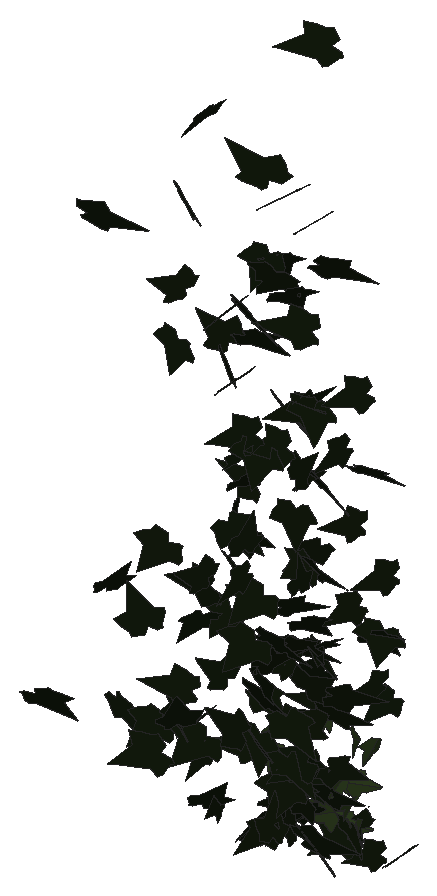
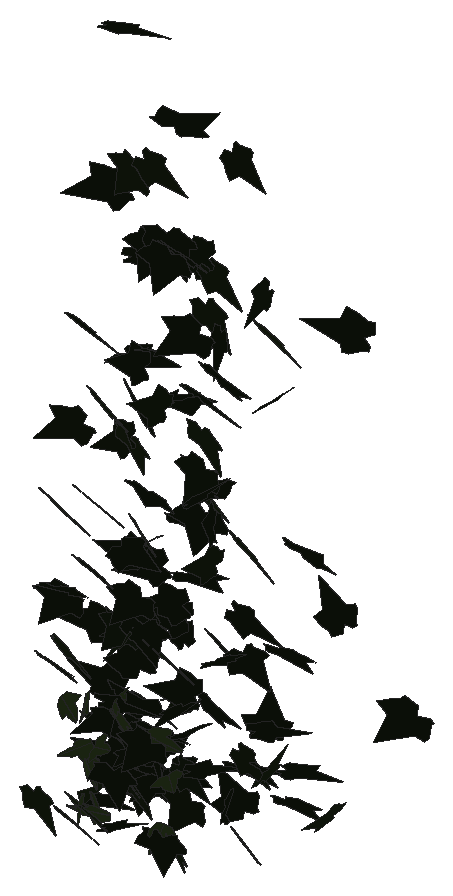
# SketchUp Ruby script. Lengths in inches.
U = 1.inch
M = Sketchup.active_model
def pt(a) = Geom::Point3d.new(a.map { |v| v * U })
def face(e, loops, mat)
  f = e.add_face(loops[0].map { |a| pt(a) })
  loops[1..].each { |l| e.add_face(l.map { |a| pt(a) }).erase! }
  f.material = f.back_material = mat if mat
  f
end
# faces: each face lists its corners as indices into pts; further lists are holes
def faces(e, pts, list, mat = nil) = list.each { |f| face(e, (f[0].is_a?(Array) ? f : [f]).map { |l| l.map { |i| pts[i] } }, mat) }
# xy, xz, yz: faces in a plane at the given z, y or x. An outline is a flat list of corners, or four numbers for a rectangle; further outlines are holes
def ring(l) = l.size == 4 ? [[l[0], l[1]], [l[2], l[1]], [l[2], l[3]], [l[0], l[3]]] : l.each_slice(2).to_a
def flat(e, list, mat, &to3) = list.each { |f| face(e, (f[0].is_a?(Array) ? f : [f]).map { |l| ring(l).map { |u, v| to3.(u, v) } }, mat) }
def xy(e, z, list, mat = nil) = flat(e, list, mat) { |x, y| [x, y, z] }
def xz(e, y, list, mat = nil) = flat(e, list, mat) { |x, z| [x, y, z] }
def yz(e, x, list, mat = nil) = flat(e, list, mat) { |y, z| [x, y, z] }
def lines(e, pts, list) = list.each { |a, b| e.add_line(pt(pts[a]), pt(pts[b])) }
# prism: a flat outline (further loops are holes) pulled along v
def prism(e, loops, v, mat = nil)
  f = face(e, loops, mat); d = Geom::Vector3d.new(v.map { |x| x * U })
  f.pushpull(f.normal.samedirection?(d) ? d.length : -d.length)
end
def box(e, o, s, mat = nil) = prism(e, [[o, [o[0] + s[0], o[1], o[2]], [o[0] + s[0], o[1] + s[1], o[2]], [o[0], o[1] + s[1], o[2]]]], [0, 0, s[2]], mat)
def at(x, y, z, deg = 0) = Geom::Transformation.translation(pt([x, y, z])) * Geom::Transformation.rotation(ORIGIN, Z_AXIS, deg.degrees)
def axes(o, x, y, z) = Geom::Transformation.new([*x, 0, *y, 0, *z, 0, *pt(o).to_a, 1])
def part(name) = M.definitions.add(name)
# library, detail: a bought-in or finely detailed component or shape, given as its bounding box
def library(name, o, s) = part(name).tap { |d| box(d.entities, o, s) }
def detail(e, o, s) = box(e.add_group.entities, o, s)
def put(e, d, t, mat = nil) = e.add_instance(d, t).tap { |i| i.material = mat if mat }
def group(e, t, mat = nil) = e.add_group.tap { |g| g.transformation = t; g.material = mat if mat }.entities
root = M.entities
M.materials.add("1026 AP 7946 SUNNY SIDE UP").color = [254, 231, 186]
M.materials.add("efeu1").color = [18, 25, 13]
M.materials.add("efeu2").color = [43, 57, 29]
c1 = part("ivyleaf_9")
p = [[1.54,2.16,1.25],[1.36,2.04,1.19],[-0.21,0.99,0.68],[-0.71,1.11,0.82],[-0.85,0.86,0.67],[-0.8,0.17,0.21],
  [-0.9,-0.01,0.1],[-0.67,-0.16,-0.02],[-0.08,-0.08,-0.05],[-0.03,-0.6,-0.4],[0.65,-0.88,-0.66],[0.83,-0.6,-0.49],
  [1.29,-0.42,-0.43],[1.8125,-0.07,-0.26],[1.21,0.44,0.15]]
faces(c1.entities,p,[[0,1,2,3,4,5,6,7,8,9,10,11,12,13,14]],"efeu1")
c2 = part("ivyleaf_10")
p = [[0,0.5,-0.03],[-0.0625,2.02,-0.43],[-0.19,2.01,-0.46],[-0.54,1.05,-0.29],[-0.52,0.625,-0.18],[-0.83,0.76,-0.28],
  [-1.16,0.64,-0.33],[-1.15,0.33,-0.24],[-0.77,-0.39,0.02],[-0.3,-0.51,0.16],[0.04,-0.48,0.23],[-0.02,2.01,-0.4375],
  [-0.06,2.01,-0.43],[0.04,-0.49,0.23],[0.67,-0.49,0.14],[1.38,0.36,-0.2],[1.375,0.51,-0.24],[0.81,0.65,-0.19],
  [0.62,0.59,-0.15],[0.6,1.09,-0.28],[0.5,1.23,-0.31]]
faces(c2.entities,p,[[0,1,2,3,4,5,6,7,8,9,10],[11,12,0,13,14,15,16,17,18,19,20]],"efeu2")
put(root,c1,axes([88.35,210.79,309.8125],[0.40505,-0.04361,0.36592],[0.56374,-0.08431,-0.26046],[0.15951,0.4087,-0.00867]),"1026 AP 7946 SUNNY SIDE UP")
put(root,c1,axes([89.35,207.07,295.36],[0.64023,0.15949,0.07493],[0.1307,-0.00845,-0.43669],[-0.26364,0.38312,-0.03454]),"1026 AP 7946 SUNNY SIDE UP")
put(root,c1,axes([89.51,210.67,293.62],[0.33265,-0.3478,-0.06127],[-0.00599,0.05837,-0.4257],[0.59711,0.19435,0.02986]),"1026 AP 7946 SUNNY SIDE UP")
put(root,c1,axes([90.67,211.54,299.03],[-0.62378,-0.1104,-0.03038],[0.06307,-0.03056,-0.40897],[0.1823,-0.36718,0.03755]),"1026 AP 7946 SUNNY SIDE UP")
put(root,c1,axes([90.63,208.78,298.75],[0.37595,0.32286,0.16484],[-0.18086,-0.10816,0.41679],[0.57645,-0.24449,0.02326]),"1026 AP 7946 SUNNY SIDE UP")
put(root,c1,axes([91.16,210.62,293.51],[-0.60289,-0.11549,0.01814],[-0.01057,-0.04023,-0.39849],[0.19826,-0.35335,0.03392]),"1026 AP 7946 SUNNY SIDE UP")
put(root,c1,axes([90.91,211.92,310.875],[0.49161,-0.16259,-0.24472],[-0.33845,0.10746,-0.35405],[0.3308,0.35158,0.00145]),"1026 AP 7946 SUNNY SIDE UP")
put(root,c1,axes([92.09,210.57,308.67],[-0.32947,0.31868,0.18492],[-0.23943,0.10907,-0.39308],[-0.56322,-0.23279,0.05893]),"1026 AP 7946 SUNNY SIDE UP")
put(root,c1,axes([91.61,210.9,306.55],[-0.14068,-0.35132,0.18544],[-0.04585,-0.17619,-0.38866],[0.66684,-0.08623,0.0124]),"1026 AP 7946 SUNNY SIDE UP")
put(root,c1,axes([92.28,209.15,293.47],[-0.54582,-0.12194,0.24605],[-0.3373,-0.12463,-0.36761],[0.28879,-0.37604,0.03568]),"1026 AP 7946 SUNNY SIDE UP")
put(root,c1,axes([92.07,211.68,292.41],[-0.48303,0.0833,-0.21493],[0.30168,-0.10429,-0.31575],[-0.21537,-0.33291,0.03974]),"1026 AP 7946 SUNNY SIDE UP")
put(root,c1,axes([92.47,210.33,295.18],[-0.31833,-0.00367,0.34467],[-0.52272,-0.10696,-0.19479],[0.15992,-0.35694,0.0494]),"1026 AP 7946 SUNNY SIDE UP")
put(root,c1,axes([92.02,210.6,293.96],[0.2802,-0.33926,-0.16995],[0.14409,-0.13013,0.40164],[-0.61607,-0.18474,0.01664]),"1026 AP 7946 SUNNY SIDE UP")
put(root,c1,axes([92.5,211.39,314.59],[-0.25235,0.27953,-0.28675],[0.14937,-0.25899,-0.34068],[-0.6444,-0.1695,0.03333]),"1026 AP 7946 SUNNY SIDE UP")
put(root,c1,axes([93.125,210.47,298.9],[-0.1617,0.01914,-0.41463],[-0.62963,-0.1217,0.08947],[-0.19346,0.38007,0.05539]),"1026 AP 7946 SUNNY SIDE UP")
put(root,c1,axes([92.81,210.56,297.71],[-0.00773,0.25127,-0.29953],[0.02589,-0.28273,-0.2729],[-0.642,-0.01443,-0.0074]),"1026 AP 7946 SUNNY SIDE UP")
put(root,c1,axes([93.17,211.3,306.93],[-0.08552,0.21206,0.37198],[-0.40306,0.2658,-0.20851],[-0.55633,-0.22517,0.09388]),"1026 AP 7946 SUNNY SIDE UP")
put(root,c1,axes([92.94,210.54,294.39],[-0.30718,0.25629,-0.20111],[0.11929,-0.18244,-0.33557],[-0.52952,-0.18978,0.04107]),"1026 AP 7946 SUNNY SIDE UP")
put(root,c1,axes([93.12,210.28,293.81],[-0.63395,-0.18201,0.03387],[-0.02398,-0.04835,-0.44366],[0.31341,-0.37187,0.03458]),"1026 AP 7946 SUNNY SIDE UP")
put(root,c1,axes([92.86,209.33,294.64],[0.4081,0.18786,0.28022],[-0.38447,-0.12943,0.32339],[0.38422,-0.32905,0.02597]),"1026 AP 7946 SUNNY SIDE UP")
put(root,c1,axes([93.51,207.04,299.23],[-0.67509,0.05875,-0.1237],[-0.18899,0.0409,0.43023],[0.11493,0.41232,-0.01913]),"1026 AP 7946 SUNNY SIDE UP")
put(root,c1,axes([93.16,211.38,297.73],[-0.31473,-0.29135,0.1333],[-0.06955,-0.12542,-0.37],[0.53593,-0.18737,0.03027]),"1026 AP 7946 SUNNY SIDE UP")
put(root,c1,axes([94.21,209,300.21],[-0.357,0.312,0.16237],[-0.16064,0.1141,-0.40096],[-0.56346,-0.23021,0.01144]),"1026 AP 7946 SUNNY SIDE UP")
put(root,c1,axes([93.57,209.68,291.99],[0.46659,0.25463,0.09948],[-0.14749,-0.03761,0.39926],[0.43383,-0.28664,0.02875]),"1026 AP 7946 SUNNY SIDE UP")
put(root,c1,axes([94.28,211.06,293.57],[-0.31836,-0.04355,0.33102],[-0.44932,-0.17038,-0.19959],[0.28298,-0.31952,0.0555]),"1026 AP 7946 SUNNY SIDE UP")
put(root,c1,axes([94.02,210.48,301.42],[-0.00216,-0.00823,0.43714],[0.20849,0.38953,0.01425],[-0.66139,0.12282,0.00306]),"1026 AP 7946 SUNNY SIDE UP")
put(root,c1,axes([93.89,210.03,292.07],[0.01141,-0.15424,-0.34654],[0.38309,-0.24735,0.12856],[-0.46903,-0.20578,0.09658]),"1026 AP 7946 SUNNY SIDE UP")
put(root,c1,axes([94.26,211.18,302.47],[-0.10473,-0.37314,-0.06699],[0.02257,-0.06059,0.40332],[-0.64055,0.05887,0.02517]),"1026 AP 7946 SUNNY SIDE UP")
put(root,c1,axes([94.27,209.82,307.33],[0.39042,-0.11108,-0.3503],[-0.5211,0.11097,-0.27099],[0.26421,0.38301,-0.01684]),"1026 AP 7946 SUNNY SIDE UP")
put(root,c1,axes([94.68,209.34,296.8125],[-0.22476,0.25202,0.28839],[-0.26401,0.21756,-0.3004],[-0.56335,-0.2025,0.02572]),"1026 AP 7946 SUNNY SIDE UP")
put(root,c1,axes([94.67,209.76,309.32],[-0.29723,0.30615,-0.21559],[0.10562,-0.19955,-0.37805],[-0.61682,-0.18169,0.03915]),"1026 AP 7946 SUNNY SIDE UP")
put(root,c1,axes([94.75,210.04,304.08],[-0.14315,0.38325,0.09427],[-0.06269,0.07682,-0.41855],[-0.66274,-0.09005,0.01923]),"1026 AP 7946 SUNNY SIDE UP")
put(root,c1,axes([94.07,210.38,300.1],[0.41419,-0.30856,0.10071],[0.07029,-0.09208,-0.42165],[0.54512,0.24633,-0.02216]),"1026 AP 7946 SUNNY SIDE UP")
put(root,c1,axes([94.49,210.32,303.06],[0.25798,0.33484,0.1589],[0.13227,0.12263,-0.39144],[-0.60448,0.16974,-0.01784]),"1026 AP 7946 SUNNY SIDE UP")
put(root,c1,axes([95.04,209.6,294.95],[-0.38704,0.00442,-0.35394],[-0.561,0.01157,0.24428],[0.02043,0.40148,0.00246]),"1026 AP 7946 SUNNY SIDE UP")
put(root,c1,axes([94.39,210.75,307.75],[0.58515,0.17168,0.13315],[0.19264,0.04603,-0.41152],[-0.30135,0.36279,-0.00452]),"1026 AP 7946 SUNNY SIDE UP")
put(root,c1,axes([94.68,210.08,301.43],[0.53247,0.18753,-0.15731],[-0.19567,-0.09774,-0.39184],[-0.35687,0.33339,-0.01987]),"1026 AP 7946 SUNNY SIDE UP")
put(root,c1,axes([95.05,211.03,290.97],[-0.24199,0.03498,-0.35985],[-0.49635,0.17113,0.15401],[0.28918,0.323,-0.0368]),"1026 AP 7946 SUNNY SIDE UP")
put(root,c1,axes([94.82,211.77,291.48],[0.36631,0.21053,-0.16052],[-0.16655,-0.11783,-0.32404],[-0.40885,0.23663,-0.01181]),"1026 AP 7946 SUNNY SIDE UP")
put(root,c2,axes([94.78,211.54,293.41],[0.22873,0.29279,-0.13915],[-0.06439,-0.12959,-0.34631],[-0.54265,0.13879,-0.01756]),"1026 AP 7946 SUNNY SIDE UP")
put(root,c1,axes([94.83,211.16,310.5],[-0.56283,-0.10998,-0.19496],[0.34668,-0.07901,-0.35084],[0.09346,-0.36923,0.1273]),"1026 AP 7946 SUNNY SIDE UP")
put(root,c1,axes([95.36,209.8,305.13],[-0.63491,0.15895,0.08712],[-0.14945,-0.00531,-0.43318],[-0.26191,-0.3823,0.03598]),"1026 AP 7946 SUNNY SIDE UP")
put(root,c1,axes([94.69,211.09,295.55],[0.13833,-0.28208,-0.24444],[-0.016,0.22856,-0.30773],[0.61193,0.06974,0.04721]),"1026 AP 7946 SUNNY SIDE UP")
put(root,c1,axes([94.96,211.28,310.34],[0.37038,0.32602,0.01366],[0.03741,-0.00453,-0.41945],[-0.55236,0.2183,-0.01925]),"1026 AP 7946 SUNNY SIDE UP")
put(root,c1,axes([94.81,209.38,302.11],[0.0867,-0.20404,-0.38713],[-0.06738,0.35759,-0.21866],[0.69765,0.05989,0.027]),"1026 AP 7946 SUNNY SIDE UP")
put(root,c2,axes([95.35,211.58,294.55],[0.21827,0.15991,-0.30184],[-0.428,-0.1447,-0.21144],[-0.35066,0.27616,0.07019]),"1026 AP 7946 SUNNY SIDE UP")
put(root,c2,axes([95.06,211.5,291.55],[-0.199,-0.27359,-0.20013],[0.1675,0.15653,-0.31537],[0.53342,-0.15122,0.02437]),"1026 AP 7946 SUNNY SIDE UP")
put(root,c1,axes([94.98,210.59,294.39],[-0.14677,-0.39406,0.07336],[0.02204,-0.07807,-0.43189],[0.68017,-0.0825,0.02982]),"1026 AP 7946 SUNNY SIDE UP")
put(root,c1,axes([95.46,208.95,307.47],[-0.17999,0.38931,-0.09475],[0.0238,-0.09314,-0.43312],[-0.67927,-0.10642,0.00993]),"1026 AP 7946 SUNNY SIDE UP")
put(root,c1,axes([95.64,210.13,313.875],[0.08829,0.12375,0.42573],[-0.6964,0.07519,0.03357],[-0.10562,-0.39231,0.1345]),"1026 AP 7946 SUNNY SIDE UP")
put(root,c1,axes([94.67,210.64,295.74],[0.48118,-0.18203,0.25205],[0.30577,-0.15797,-0.36151],[0.40615,0.33458,-0.02646]),"1026 AP 7946 SUNNY SIDE UP")
put(root,c1,axes([95.15,211.96,294.58],[0.54043,0.16246,0.00292],[0.02063,-0.02247,-0.38198],[-0.27502,0.31757,-0.02291]),"1026 AP 7946 SUNNY SIDE UP")
put(root,c1,axes([94.96,209.61,309.53],[0.54959,-0.23504,0.1061],[0.10894,-0.08502,-0.42829],[0.4212,0.32868,-0.02767]),"1026 AP 7946 SUNNY SIDE UP")
put(root,c1,axes([95.66,210.51,310.45],[0.35833,0.13459,-0.34297],[-0.45301,-0.18048,-0.27047],[-0.38207,0.34021,-0.00097]),"1026 AP 7946 SUNNY SIDE UP")
put(root,c1,axes([95.4,209.82,291.63],[0.28304,0.33113,0.1889],[0.13305,0.15325,-0.39477],[-0.61938,0.18424,0.00152]),"1026 AP 7946 SUNNY SIDE UP")
put(root,c1,axes([95.96,210.95,297.1],[-0.54413,0.2458,0.04579],[-0.10667,-0.01746,-0.42911],[-0.40894,-0.3225,0.051]),"1026 AP 7946 SUNNY SIDE UP")
put(root,c1,axes([95.09,211.48,305.36],[0.39573,-0.27888,0.19115],[0.16185,-0.1572,-0.39043],[0.54182,0.25064,-0.02298]),"1026 AP 7946 SUNNY SIDE UP")
put(root,c1,axes([95.76,208.9,301.83],[-0.46951,0.2629,-0.12032],[-0.12898,0.0881,0.40959],[0.4703,0.28662,-0.00779]),"1026 AP 7946 SUNNY SIDE UP")
put(root,c1,axes([95.92,211.14,313.07],[-0.34268,0.26206,-0.23595],[0.02122,-0.25365,-0.33356],[-0.58463,-0.16281,0.1262]),"1026 AP 7946 SUNNY SIDE UP")
put(root,c1,axes([95.67,209.79,304.69],[-0.34234,-0.34354,-0.01321],[0.0411,-0.00511,-0.42581],[0.58189,-0.20176,0.0223]),"1026 AP 7946 SUNNY SIDE UP")
put(root,c1,axes([95.92,209.57,292.47],[-0.28818,0.2543,-0.25059],[0.16828,-0.21783,-0.32876],[-0.56606,-0.19422,0.02984]),"1026 AP 7946 SUNNY SIDE UP")
put(root,c1,axes([95.93,209.11,298.59],[-0.5587,-0.23379,0.0543],[-0.04548,-0.05489,-0.43185],[0.40468,-0.32894,0.02643]),"1026 AP 7946 SUNNY SIDE UP")
put(root,c1,axes([96.1,210.375,304.71],[-0.29778,-0.11327,0.3473],[-0.36446,-0.25033,-0.22038],[0.45845,-0.27259,0.05039]),"1026 AP 7946 SUNNY SIDE UP")
put(root,c1,axes([96.04,211.15,297.76],[0.24108,0.26625,-0.21466],[-0.18017,-0.17445,-0.32533],[-0.5401,0.17704,0.01271]),"1026 AP 7946 SUNNY SIDE UP")
put(root,c1,axes([96.1,208.5,301.17],[-0.53534,0.18536,-0.20246],[0.24953,-0.12655,-0.39201],[-0.37743,-0.34658,0.028]),"1026 AP 7946 SUNNY SIDE UP")
put(root,c1,axes([96.12,211.95,300.64],[-0.08308,0.09831,-0.38832],[0.05864,-0.36434,-0.11541],[-0.63736,-0.04634,0.04]),"1026 AP 7946 SUNNY SIDE UP")
put(root,c1,axes([95.78,209.4,295.03],[0.55655,-0.15769,-0.17424],[-0.2563,0.05659,-0.38844],[0.28351,0.36071,-0.00911]),"1026 AP 7946 SUNNY SIDE UP")
put(root,c1,axes([96.41,212.13,317.77],[-0.57652,-0.01129,0.25447],[-0.37714,-0.13404,-0.3483],[0.14543,-0.39236,0.10555]),"1026 AP 7946 SUNNY SIDE UP")
put(root,c1,axes([95.75,209.6875,296.77],[-0.05871,-0.02523,0.40491],[0.17939,-0.36571,-0.02086],[0.61854,0.10367,0.04449]),"1026 AP 7946 SUNNY SIDE UP")
put(root,c1,axes([95.76,209.67,297.45],[0.20527,0.06969,0.41453],[0.4965,0.25358,-0.14346],[-0.4444,0.3155,0.0312]),"1026 AP 7946 SUNNY SIDE UP")
put(root,c1,axes([95.55,210.1,298.14],[0.54748,-0.07235,0.19968],[0.29152,-0.08482,-0.35253],[0.17711,0.36327,-0.03699]),"1026 AP 7946 SUNNY SIDE UP")
put(root,c1,axes([96.26,209.0625,300.29],[-0.64963,-0.13181,-0.01677],[0.04527,-0.03482,-0.43151],[0.22039,-0.38136,0.03919]),"1026 AP 7946 SUNNY SIDE UP")
put(root,c1,axes([95.94,211.1,302.2],[-0.43671,-0.13434,-0.27347],[0.45284,0.01396,-0.29733],[0.18001,-0.36104,0.08452]),"1026 AP 7946 SUNNY SIDE UP")
put(root,c1,axes([96.53,210.79,293.6],[-0.09617,0.2777,0.28968],[-0.33232,0.21163,-0.27721],[-0.56318,-0.17231,0.11411]),"1026 AP 7946 SUNNY SIDE UP")
put(root,c1,axes([96.27,209.43,292.23],[-0.03168,0.04599,-0.43966],[0.12861,-0.40435,-0.05774],[-0.69063,-0.07741,0.00942]),"1026 AP 7946 SUNNY SIDE UP")
put(root,c1,axes([96.11,210.42,309.96],[0.37436,0.33042,0.04423],[0.05488,0.02289,-0.42471],[-0.56174,0.22244,-0.01201]),"1026 AP 7946 SUNNY SIDE UP")
put(root,c1,axes([96.26,211.28,300.3125],[-0.31037,-0.16485,0.27811],[-0.16161,-0.25951,-0.24962],[0.49989,-0.18625,0.09197]),"1026 AP 7946 SUNNY SIDE UP")
put(root,c1,axes([96.71,211.99,295.39],[-0.38276,0.06279,0.28868],[-0.46227,0.00641,-0.24604],[-0.07696,-0.35081,0.04211]),"1026 AP 7946 SUNNY SIDE UP")
put(root,c1,axes([96.49,212.23,291.47],[-0.34411,-0.06342,0.26405],[-0.30666,-0.18778,-0.21257],[0.30663,-0.25898,0.08374]),"1026 AP 7946 SUNNY SIDE UP")
put(root,c1,axes([96.05,211.33,296.49],[0.56365,0.18027,0.10105],[-0.17918,0.00334,0.40071],[0.29317,-0.34454,0.05063]),"1026 AP 7946 SUNNY SIDE UP")
put(root,c1,axes([95.89,210.95,297.63],[0.52122,0.07724,0.2231],[0.34796,0.03445,-0.33815],[-0.14161,0.36892,-0.00972]),"1026 AP 7946 SUNNY SIDE UP")
put(root,c1,axes([96.21,210.15,292.28],[0.28229,0.27591,0.23988],[0.2432,0.17004,-0.34113],[-0.54799,0.21759,-0.02782]),"1026 AP 7946 SUNNY SIDE UP")
put(root,c1,axes([96.49,211.95,293.17],[0.23534,0.27674,-0.13947],[-0.10566,-0.11856,-0.33302],[-0.51106,0.15195,0.00462]),"1026 AP 7946 SUNNY SIDE UP")
put(root,c2,axes([96.46,211.86,295.03],[0.43618,-0.2116,-0.06495],[-0.10715,0.0141,-0.35482],[0.35666,0.26302,-0.02717]),"1026 AP 7946 SUNNY SIDE UP")
put(root,c2,axes([96.3,212,295.52],[-0.09123,-0.10261,0.34642],[0.22769,-0.30875,-0.08495],[0.53172,0.11461,0.09581]),"1026 AP 7946 SUNNY SIDE UP")
put(root,c1,axes([96.45,210.66,292.4375],[0.3233,0.28286,-0.09249],[-0.06097,-0.08428,-0.36581],[-0.50023,0.19309,-0.01519]),"1026 AP 7946 SUNNY SIDE UP")
put(root,c1,axes([96.7,210.89,303.58],[-0.06087,0.34087,0.1853],[-0.10142,0.16223,-0.3624],[-0.63756,-0.05835,0.03996]),"1026 AP 7946 SUNNY SIDE UP")
put(root,c1,axes([96.17,211.02,294.86],[-0.28083,0.07371,0.34677],[0.54272,-0.05895,0.18891],[0.14717,0.35804,-0.03495]),"1026 AP 7946 SUNNY SIDE UP")
put(root,c1,axes([96.3,211.01,298.54],[0.4291,0.24727,0.10508],[0.13593,0.05374,-0.37738],[-0.42859,0.26461,-0.01449]),"1026 AP 7946 SUNNY SIDE UP")
put(root,c1,axes([96.14,210.28,299.31],[0.36415,0.12019,0.31026],[0.40454,0.163,-0.26036],[-0.34262,0.3202,0.02234]),"1026 AP 7946 SUNNY SIDE UP")
put(root,c1,axes([96.74,210.82,292.34],[-0.18836,0.33194,-0.02176],[-0.00602,-0.02716,-0.37486],[-0.56501,-0.11037,0.01125]),"1026 AP 7946 SUNNY SIDE UP")
put(root,c1,axes([96.66,210.36,300.14],[0.12977,0.09567,0.37912],[-0.08073,0.36005,-0.08845],[-0.61538,-0.02706,0.09155]),"1026 AP 7946 SUNNY SIDE UP")
put(root,c1,axes([96.34,211.47,297.55],[0.36717,-0.23728,-0.19127],[-0.20081,0.12973,-0.34192],[0.45907,0.24653,0.00342]),"1026 AP 7946 SUNNY SIDE UP")
put(root,c1,axes([96.07,211.48,300.16],[0.31579,-0.15924,0.2767],[0.3588,-0.15301,-0.26383],[0.37407,0.28119,0.01947]),"1026 AP 7946 SUNNY SIDE UP")
put(root,c1,axes([96.66,211.6875,292.89],[-0.02089,-0.11965,-0.35453],[0.14372,-0.32106,0.11691],[-0.57762,-0.07555,0.04191]),"1026 AP 7946 SUNNY SIDE UP")
put(root,c1,axes([96.375,210.79,306],[0.15237,0.0434,0.40009],[0.42544,0.27888,-0.09537],[-0.47504,0.26367,0.04292]),"1026 AP 7946 SUNNY SIDE UP")
put(root,c1,axes([96.89,210.69,306.16],[-0.08514,-0.09958,-0.40381],[-0.09635,-0.37307,0.10871],[-0.65303,0.06803,0.03661]),"1026 AP 7946 SUNNY SIDE UP")
put(root,c1,axes([96.54,211.32,297.625],[0.31546,0.24897,0.20131],[0.1143,0.1779,-0.3266],[-0.51377,0.19245,0.05095]),"1026 AP 7946 SUNNY SIDE UP")
put(root,c1,axes([96.64,209.84,293.625],[-0.56373,-0.15293,-0.14398],[0.25644,-0.01797,-0.38339],[0.22852,-0.35709,0.07504]),"1026 AP 7946 SUNNY SIDE UP")
put(root,c1,axes([96.41,210.91,293.35],[-0.01902,-0.20664,-0.30084],[0.08713,0.2744,-0.2165],[0.58194,-0.04783,0.02258]),"1026 AP 7946 SUNNY SIDE UP")
put(root,c1,axes([96.84,210.87,294.03],[0.35656,0.00656,-0.3069],[-0.47885,-0.0596,-0.2235],[-0.08813,0.35041,-0.02723]),"1026 AP 7946 SUNNY SIDE UP")
put(root,c1,axes([96.68,210.72,312.3],[0.25649,0.27862,0.28835],[0.09973,0.2654,-0.33001],[-0.64591,0.15162,0.06355]),"1026 AP 7946 SUNNY SIDE UP")
put(root,c1,axes([97.13,210.22,309.12],[-0.39439,-0.01729,0.35897],[-0.5332,-0.13359,-0.24208],[0.2024,-0.38563,0.06173]),"1026 AP 7946 SUNNY SIDE UP")
put(root,c1,axes([96.75,209.94,292.09],[-0.07535,-0.00877,0.38873],[-0.24856,-0.33445,-0.03247],[0.56445,-0.14845,0.03759]),"1026 AP 7946 SUNNY SIDE UP")
put(root,c1,axes([97.02,209.96,293.26],[0.28609,-0.012,-0.3842],[-0.60186,-0.06723,-0.17686],[-0.0948,0.39059,-0.03663]),"1026 AP 7946 SUNNY SIDE UP")
put(root,c1,axes([96.81,208.94,292.37],[-0.25763,-0.19958,0.3457],[0.33299,0.25977,0.27205],[-0.55609,0.24801,0.00275]),"1026 AP 7946 SUNNY SIDE UP")
put(root,c1,axes([96.6,210.33,303.88],[-0.14686,0.27246,0.30491],[0.11021,-0.27407,0.30179],[0.65553,0.10712,0.01757]),"1026 AP 7946 SUNNY SIDE UP")
put(root,c1,axes([97.22,209.97,294.53],[-0.66292,0.05764,-0.02169],[0.02534,-0.04202,-0.42109],[-0.10102,-0.38882,0.03668]),"1026 AP 7946 SUNNY SIDE UP")
put(root,c2,axes([97.23,211,292.36],[0.36701,-0.08888,-0.27398],[-0.41471,0.07411,-0.2486],[0.19445,0.32581,-0.01307]),"1026 AP 7946 SUNNY SIDE UP")
put(root,c1,axes([96.89,210.78,306.24],[-0.19678,-0.37348,-0.03143],[0.03053,0.02005,-0.41821],[0.63463,-0.11677,0.01037]),"1026 AP 7946 SUNNY SIDE UP")
put(root,c1,axes([96.7,209.82,294.5],[0.05033,-0.38077,-0.10511],[0.22712,0.0977,-0.38032],[0.6255,-0.00484,0.14655]),"1026 AP 7946 SUNNY SIDE UP")
put(root,c1,axes([96.7,211.03,303.64],[0.52788,-0.21647,0.06681],[0.05783,-0.06479,-0.40498],[0.37941,0.31106,-0.03123]),"1026 AP 7946 SUNNY SIDE UP")
put(root,c1,axes([96.77,210.62,296.58],[-0.15237,0.04355,0.37468],[0.41318,-0.25289,0.09715],[0.43192,0.25728,0.03924]),"1026 AP 7946 SUNNY SIDE UP")
put(root,c1,axes([97.68,211.92,301.93],[-0.49449,0.21486,0.08339],[-0.14859,0.00682,-0.38434],[-0.35665,-0.30074,0.04451]),"1026 AP 7946 SUNNY SIDE UP")
put(root,c1,axes([97.78,211.88,291.65],[-0.19319,0.28073,0.18304],[-0.24672,0.11613,-0.30284],[-0.45895,-0.18059,0.08575]),"1026 AP 7946 SUNNY SIDE UP")
put(root,c1,axes([97.64,211.3125,304.8],[-0.5513,0.16033,-0.13491],[0.16676,-0.0891,-0.38724],[-0.30587,-0.33755,0.03204]),"1026 AP 7946 SUNNY SIDE UP")
put(root,c2,axes([97.01,211.875,291.57],[0.05242,-0.12747,-0.3195],[0.54622,0.03805,0.01888],[0.04764,-0.29594,0.13509]),"1026 AP 7946 SUNNY SIDE UP")
put(root,c2,axes([97.58,211.5,291.71],[0.21705,-0.26761,-0.15761],[-0.09551,0.13239,-0.31562],[0.50674,0.13958,0.00802]),"1026 AP 7946 SUNNY SIDE UP")
put(root,c2,axes([97.51,211.43,293.4],[0.08905,0.17657,-0.30653],[-0.14312,-0.27604,-0.20105],[-0.55625,0.09929,0.00266]),"1026 AP 7946 SUNNY SIDE UP")
put(root,c1,axes([97.73,211.24,291.52],[-0.44085,-0.14949,0.164],[-0.20773,-0.09191,-0.3274],[0.27465,-0.30947,0.01562]),"1026 AP 7946 SUNNY SIDE UP")
put(root,c1,axes([97.06,210.9375,293],[0.33596,0.09409,-0.28905],[0.38873,0.14693,0.23551],[0.2939,-0.30189,0.01892]),"1026 AP 7946 SUNNY SIDE UP")
put(root,c1,axes([97.07,211.32,295.53],[0.17869,-0.09923,0.34698],[0.49496,-0.14917,-0.15175],[0.29751,0.30776,0.04407]),"1026 AP 7946 SUNNY SIDE UP")
put(root,c1,axes([97.88,211.59,299.38],[-0.58396,0.09726,-0.04696],[0.05537,-0.04954,-0.38118],[-0.17338,-0.3434,0.03641]),"1026 AP 7946 SUNNY SIDE UP")
put(root,c1,axes([97.38,208.93,296.54],[0.02216,-0.3211,-0.27481],[0.05747,0.25262,-0.33851],[0.69104,-0.01071,0.03696]),"1026 AP 7946 SUNNY SIDE UP")
put(root,c2,axes([97.77,211.49,292.74],[0.06617,-0.33281,0.03487],[0.0031,-0.03694,-0.35924],[0.56842,0.03894,-0.0021]),"1026 AP 7946 SUNNY SIDE UP")
put(root,c1,axes([97.54,210.79,294.1],[0.08827,0.01057,-0.38072],[-0.04521,0.35864,0.01225],[0.60248,0.02536,0.0567]),"1026 AP 7946 SUNNY SIDE UP")
put(root,c2,axes([97.82,211.76,291.67],[-0.18463,0.29689,0.12708],[-0.14457,0.08979,-0.33362],[-0.52066,-0.13021,0.04757]),"1026 AP 7946 SUNNY SIDE UP")
put(root,c2,axes([97.83,211.5,294.85],[0.14252,-0.17027,-0.31729],[0.00975,0.30366,-0.18219],[0.57687,0.03693,0.08147]),"1026 AP 7946 SUNNY SIDE UP")
put(root,c1,axes([97.65,211.52,291.82],[0.11247,-0.30626,0.12636],[0.06149,-0.11694,-0.33692],[0.55625,0.07485,0.0117]),"1026 AP 7946 SUNNY SIDE UP")
put(root,c1,axes([97.5,210.45,311.36],[0.55505,0.09132,0.26371],[0.41013,0.04504,-0.36233],[-0.17027,0.40617,-0.01309]),"1026 AP 7946 SUNNY SIDE UP")
put(root,c2,axes([97.84,211.54,293.35],[0.00867,-0.13725,-0.33693],[0.37176,0.24155,-0.10622],[0.44525,-0.19901,0.09525]),"1026 AP 7946 SUNNY SIDE UP")
put(root,c1,axes([98.47,211.21,307.01],[-0.6083,0.14161,0.03661],[-0.07251,-0.02041,-0.41113],[-0.23568,-0.35922,0.03198]),"1026 AP 7946 SUNNY SIDE UP")
put(root,c1,axes([97.71,209.38,292.45],[0.38613,-0.29126,0.13488],[0.09077,-0.12232,-0.39593],[0.53362,0.23156,-0.03025]),"1026 AP 7946 SUNNY SIDE UP")
put(root,c1,axes([98.47,212,296.76],[-0.44144,0.23266,-0.02579],[0.00455,-0.03757,-0.37304],[-0.3976,-0.25874,0.02437]),"1026 AP 7946 SUNNY SIDE UP")
put(root,c1,axes([98.56,211.77,291.05],[-0.49636,0.16344,0.04481],[-0.08274,-0.00608,-0.35737],[-0.27327,-0.29503,0.0268]),"1026 AP 7946 SUNNY SIDE UP")
put(root,c1,axes([97.875,211.73,304.02],[0.60676,0.0539,0.12192],[0.16523,0.09621,-0.37678],[-0.13411,0.36237,0.08742]),"1026 AP 7946 SUNNY SIDE UP")
put(root,c2,axes([98.36,211.82,294.75],[-0.04065,-0.30641,0.15677],[0.03605,-0.15184,-0.32962],[0.57833,-0.01207,0.03157]),"1026 AP 7946 SUNNY SIDE UP")
put(root,c1,axes([98.21,211.9375,298.34],[0.51084,0.19106,0.03204],[0.05733,-0.00208,-0.38106],[-0.3226,0.30217,-0.01698]),"1026 AP 7946 SUNNY SIDE UP")
put(root,c1,axes([98,210.4,296.88],[0.23963,0.16526,-0.33284],[0.21182,0.29216,0.22944],[0.56235,-0.18047,0.05541]),"1026 AP 7946 SUNNY SIDE UP")
put(root,c1,axes([98.68,212.24,296.22],[-0.57141,0.00432,-0.09487],[0.14461,-0.08211,-0.35165],[-0.04241,-0.33827,0.07915]),"1026 AP 7946 SUNNY SIDE UP")
put(root,c1,axes([97.97,209.13,292.5],[0.26047,-0.0839,0.39742],[0.57462,-0.15542,-0.18901],[0.29923,0.37149,0.01703]),"1026 AP 7946 SUNNY SIDE UP")
put(root,c1,axes([98.52,212.0625,298.56],[-0.41625,-0.24093,-0.10702],[0.17894,0.02933,-0.36355],[0.40282,-0.26199,0.05091]),"1026 AP 7946 SUNNY SIDE UP")
put(root,c1,axes([99.34,211.41,301],[-0.58158,0.21666,0.00102],[-0.02864,-0.03017,-0.43282],[-0.36668,-0.34128,0.03219]),"1026 AP 7946 SUNNY SIDE UP")
put(root,c1,axes([99.47,211.82,291.35],[-0.17399,0.34535,-0.0556],[0.00874,-0.05732,-0.38628],[-0.59396,-0.10201,0.01061]),"1026 AP 7946 SUNNY SIDE UP")
